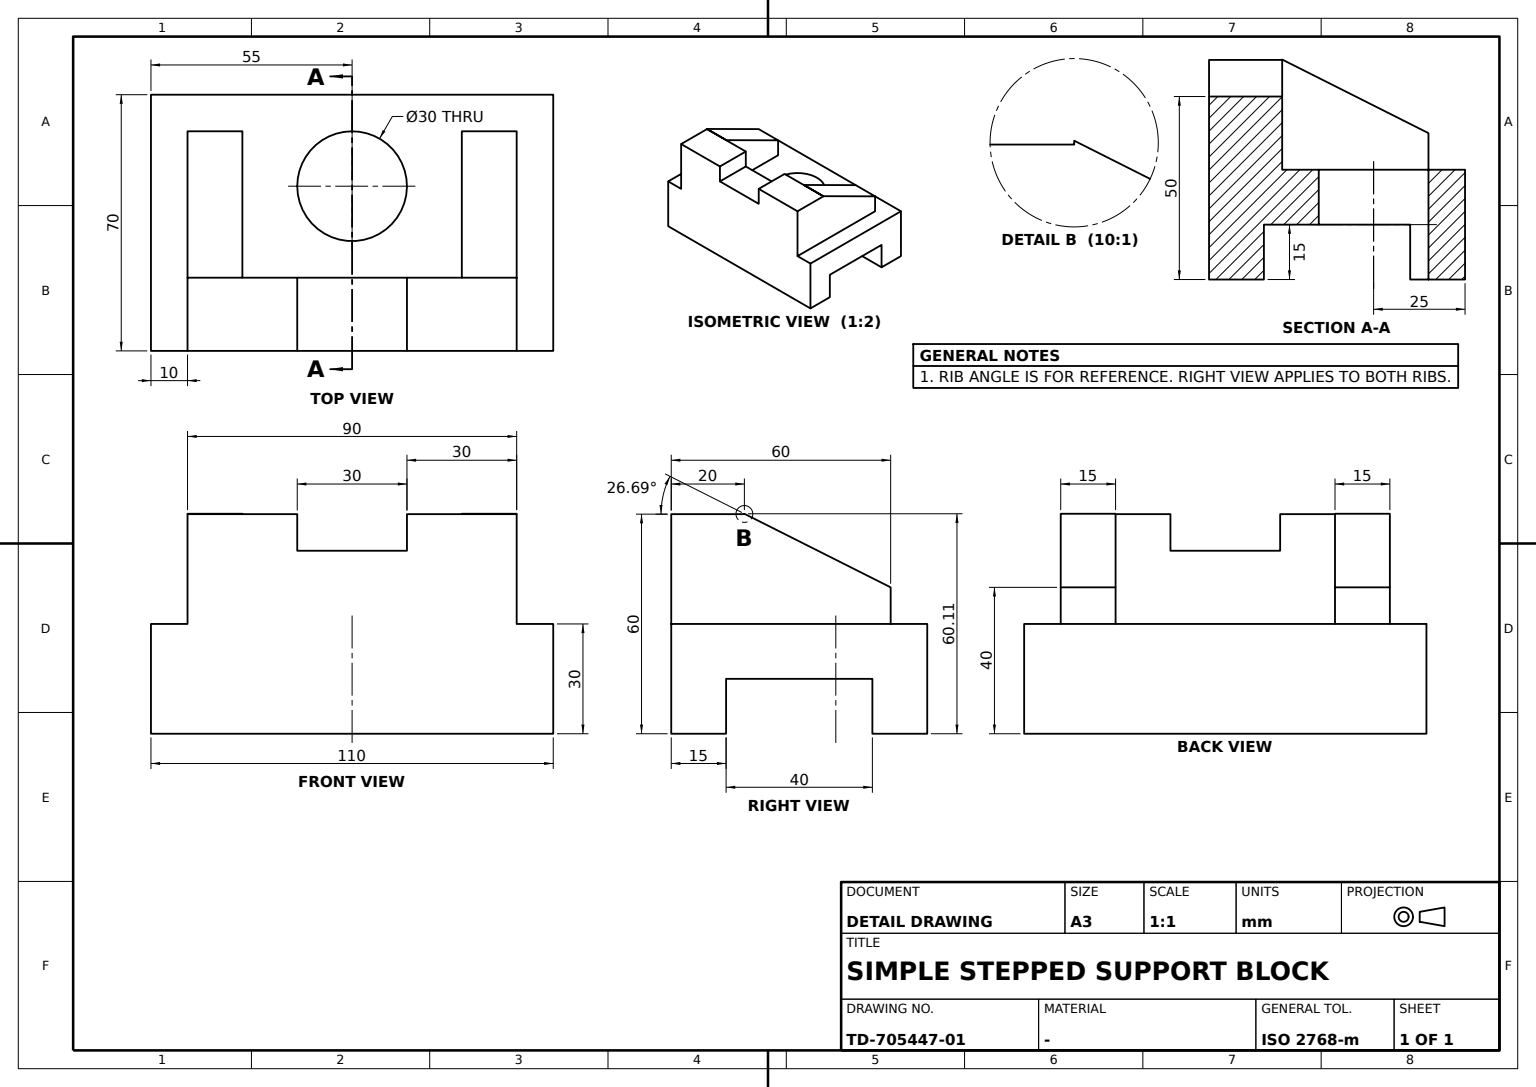
ISO-10303-21;
HEADER;
FILE_DESCRIPTION((''),'2;1');
FILE_NAME('','',(''),(''),'','','');
FILE_SCHEMA(('AUTOMOTIVE_DESIGN'));
ENDSEC;
DATA;
#1=APPLICATION_CONTEXT('');
#2=PRODUCT_CONTEXT('',#1,'mechanical');
#3=PRODUCT('','','',(#2));
#4=PRODUCT_DEFINITION_FORMATION('','',#3);
#5=PRODUCT_DEFINITION_CONTEXT('',#1,'design');
#6=PRODUCT_DEFINITION('','',#4,#5);
#7=PRODUCT_DEFINITION_SHAPE('','',#6);
#8=(LENGTH_UNIT()NAMED_UNIT(*)SI_UNIT(.MILLI.,.METRE.));
#9=(NAMED_UNIT(*)PLANE_ANGLE_UNIT()SI_UNIT($,.RADIAN.));
#10=(NAMED_UNIT(*)SI_UNIT($,.STERADIAN.)SOLID_ANGLE_UNIT());
#11=UNCERTAINTY_MEASURE_WITH_UNIT(LENGTH_MEASURE(0.005),#8,'distance_accuracy_value','');
#12=(GEOMETRIC_REPRESENTATION_CONTEXT(3)GLOBAL_UNCERTAINTY_ASSIGNED_CONTEXT((#11))GLOBAL_UNIT_ASSIGNED_CONTEXT((#8,#9,#10))REPRESENTATION_CONTEXT('',''));
#13=CARTESIAN_POINT('',(-15.,10.,7.5));
#14=VERTEX_POINT('',#13);
#15=CARTESIAN_POINT('',(0.,10.,7.5));
#16=DIRECTION('',(0.,0.,-1.));
#17=DIRECTION('',(-1.,0.,0.));
#18=AXIS2_PLACEMENT_3D('',#15,#16,#17);
#19=CIRCLE('',#18,15.);
#20=EDGE_CURVE('',#14,#14,#19,.T.);
#21=ORIENTED_EDGE('',*,*,#20,.T.);
#22=EDGE_LOOP('',(#21));
#23=FACE_BOUND('',#22,.T.);
#24=CARTESIAN_POINT('',(-55.,-35.,7.5));
#25=VERTEX_POINT('',#24);
#26=CARTESIAN_POINT('',(-45.,-35.,7.5));
#27=VERTEX_POINT('',#26);
#28=CARTESIAN_POINT('',(0.,-35.,7.5));
#29=DIRECTION('',(1.,0.,0.));
#30=VECTOR('',#29,1000.);
#31=LINE('',#28,#30);
#32=EDGE_CURVE('',#25,#27,#31,.T.);
#33=ORIENTED_EDGE('',*,*,#32,.T.);
#34=CARTESIAN_POINT('',(-45.,25.,7.5));
#35=VERTEX_POINT('',#34);
#36=DIRECTION('',(0.,1.,0.));
#37=VECTOR('',#36,1000.);
#38=LINE('',#26,#37);
#39=EDGE_CURVE('',#27,#35,#38,.T.);
#40=ORIENTED_EDGE('',*,*,#39,.T.);
#41=CARTESIAN_POINT('',(-30.,25.,7.5));
#42=VERTEX_POINT('',#41);
#43=CARTESIAN_POINT('',(0.,25.,7.5));
#44=LINE('',#43,#30);
#45=EDGE_CURVE('',#35,#42,#44,.T.);
#46=ORIENTED_EDGE('',*,*,#45,.T.);
#47=CARTESIAN_POINT('',(-30.,-15.,7.5));
#48=VERTEX_POINT('',#47);
#49=CARTESIAN_POINT('',(-30.,-35.,7.5));
#50=DIRECTION('',(0.,-1.,0.));
#51=VECTOR('',#50,1000.);
#52=LINE('',#49,#51);
#53=EDGE_CURVE('',#42,#48,#52,.T.);
#54=ORIENTED_EDGE('',*,*,#53,.T.);
#55=CARTESIAN_POINT('',(30.,-15.,7.5));
#56=VERTEX_POINT('',#55);
#57=CARTESIAN_POINT('',(0.,-15.,7.5));
#58=LINE('',#57,#30);
#59=EDGE_CURVE('',#48,#56,#58,.T.);
#60=ORIENTED_EDGE('',*,*,#59,.T.);
#61=CARTESIAN_POINT('',(30.,25.,7.5));
#62=VERTEX_POINT('',#61);
#63=CARTESIAN_POINT('',(30.,-35.,7.5));
#64=LINE('',#63,#51);
#65=EDGE_CURVE('',#62,#56,#64,.T.);
#66=ORIENTED_EDGE('',*,*,#65,.F.);
#67=CARTESIAN_POINT('',(45.,25.,7.5));
#68=VERTEX_POINT('',#67);
#69=VECTOR('',#17,1000.);
#70=LINE('',#67,#69);
#71=EDGE_CURVE('',#68,#62,#70,.T.);
#72=ORIENTED_EDGE('',*,*,#71,.F.);
#73=CARTESIAN_POINT('',(45.,-35.,7.5));
#74=VERTEX_POINT('',#73);
#75=LINE('',#73,#37);
#76=EDGE_CURVE('',#74,#68,#75,.T.);
#77=ORIENTED_EDGE('',*,*,#76,.F.);
#78=CARTESIAN_POINT('',(55.,-35.,7.5));
#79=VERTEX_POINT('',#78);
#80=EDGE_CURVE('',#74,#79,#31,.T.);
#81=ORIENTED_EDGE('',*,*,#80,.T.);
#82=CARTESIAN_POINT('',(55.,35.,7.5));
#83=VERTEX_POINT('',#82);
#84=CARTESIAN_POINT('',(55.,0.,7.5));
#85=LINE('',#84,#37);
#86=EDGE_CURVE('',#79,#83,#85,.T.);
#87=ORIENTED_EDGE('',*,*,#86,.T.);
#88=CARTESIAN_POINT('',(-55.,35.,7.5));
#89=VERTEX_POINT('',#88);
#90=CARTESIAN_POINT('',(0.,35.,7.5));
#91=LINE('',#90,#30);
#92=EDGE_CURVE('',#89,#83,#91,.T.);
#93=ORIENTED_EDGE('',*,*,#92,.F.);
#94=CARTESIAN_POINT('',(-55.,0.,7.5));
#95=LINE('',#94,#37);
#96=EDGE_CURVE('',#25,#89,#95,.T.);
#97=ORIENTED_EDGE('',*,*,#96,.F.);
#98=EDGE_LOOP('',(#33,#40,#46,#54,#60,#66,#72,#77,#81,#87,#93,#97));
#99=FACE_BOUND('',#98,.T.);
#100=AXIS2_PLACEMENT_3D('',#28,#16,#36);
#101=PLANE('',#100);
#102=ADVANCED_FACE('',(#23,#99),#101,.F.);
#103=CARTESIAN_POINT('',(-15.,-35.,27.5));
#104=VERTEX_POINT('',#103);
#105=CARTESIAN_POINT('',(-15.,-35.,37.5));
#106=VERTEX_POINT('',#105);
#107=CARTESIAN_POINT('',(-15.,-35.,-22.5));
#108=DIRECTION('',(0.,0.,1.));
#109=VECTOR('',#108,1000.);
#110=LINE('',#107,#109);
#111=EDGE_CURVE('',#104,#106,#110,.T.);
#112=ORIENTED_EDGE('',*,*,#111,.F.);
#113=CARTESIAN_POINT('',(-15.,-15.,27.5));
#114=VERTEX_POINT('',#113);
#115=LINE('',#103,#37);
#116=EDGE_CURVE('',#104,#114,#115,.T.);
#117=ORIENTED_EDGE('',*,*,#116,.T.);
#118=CARTESIAN_POINT('',(-15.,-15.,37.5));
#119=VERTEX_POINT('',#118);
#120=LINE('',#113,#109);
#121=EDGE_CURVE('',#114,#119,#120,.T.);
#122=ORIENTED_EDGE('',*,*,#121,.T.);
#123=LINE('',#105,#37);
#124=EDGE_CURVE('',#106,#119,#123,.T.);
#125=ORIENTED_EDGE('',*,*,#124,.F.);
#126=EDGE_LOOP('',(#112,#117,#122,#125));
#127=FACE_BOUND('',#126,.T.);
#128=AXIS2_PLACEMENT_3D('',#103,#17,#108);
#129=PLANE('',#128);
#130=ADVANCED_FACE('',(#127),#129,.F.);
#131=CARTESIAN_POINT('',(-45.,25.,17.5));
#132=VERTEX_POINT('',#131);
#133=CARTESIAN_POINT('',(-30.,25.,17.5));
#134=VERTEX_POINT('',#133);
#135=CARTESIAN_POINT('',(45.,25.,17.5));
#136=LINE('',#135,#30);
#137=EDGE_CURVE('',#132,#134,#136,.T.);
#138=ORIENTED_EDGE('',*,*,#137,.F.);
#139=CARTESIAN_POINT('',(-45.,-15.,37.605849));
#140=VERTEX_POINT('',#139);
#141=DIRECTION('',(0.,0.893479455,-0.449104067));
#142=VECTOR('',#141,1000.);
#143=LINE('',#139,#142);
#144=EDGE_CURVE('',#140,#132,#143,.T.);
#145=ORIENTED_EDGE('',*,*,#144,.F.);
#146=CARTESIAN_POINT('',(-30.,-15.,37.605849));
#147=VERTEX_POINT('',#146);
#148=CARTESIAN_POINT('',(45.,-15.,37.605849));
#149=LINE('',#148,#30);
#150=EDGE_CURVE('',#140,#147,#149,.T.);
#151=ORIENTED_EDGE('',*,*,#150,.T.);
#152=LINE('',#146,#142);
#153=EDGE_CURVE('',#147,#134,#152,.T.);
#154=ORIENTED_EDGE('',*,*,#153,.T.);
#155=EDGE_LOOP('',(#138,#145,#151,#154));
#156=FACE_BOUND('',#155,.T.);
#157=DIRECTION('',(0.,0.449104067,0.893479455));
#158=AXIS2_PLACEMENT_3D('',#148,#157,#141);
#159=PLANE('',#158);
#160=ADVANCED_FACE('',(#156),#159,.T.);
#161=ORIENTED_EDGE('',*,*,#92,.T.);
#162=CARTESIAN_POINT('',(55.,35.,-22.5));
#163=VERTEX_POINT('',#162);
#164=CARTESIAN_POINT('',(55.,35.,0.));
#165=VECTOR('',#16,1000.);
#166=LINE('',#164,#165);
#167=EDGE_CURVE('',#83,#163,#166,.T.);
#168=ORIENTED_EDGE('',*,*,#167,.T.);
#169=CARTESIAN_POINT('',(-55.,35.,-22.5));
#170=VERTEX_POINT('',#169);
#171=CARTESIAN_POINT('',(0.,35.,-22.5));
#172=LINE('',#171,#30);
#173=EDGE_CURVE('',#170,#163,#172,.T.);
#174=ORIENTED_EDGE('',*,*,#173,.F.);
#175=CARTESIAN_POINT('',(-55.,35.,0.));
#176=LINE('',#175,#165);
#177=EDGE_CURVE('',#89,#170,#176,.T.);
#178=ORIENTED_EDGE('',*,*,#177,.F.);
#179=EDGE_LOOP('',(#161,#168,#174,#178));
#180=FACE_BOUND('',#179,.T.);
#181=AXIS2_PLACEMENT_3D('',#90,#50,#16);
#182=PLANE('',#181);
#183=ADVANCED_FACE('',(#180),#182,.F.);
#184=CARTESIAN_POINT('',(-45.,-35.,37.5));
#185=VERTEX_POINT('',#184);
#186=CARTESIAN_POINT('',(-45.,-15.,37.5));
#187=VERTEX_POINT('',#186);
#188=LINE('',#184,#37);
#189=EDGE_CURVE('',#185,#187,#188,.T.);
#190=ORIENTED_EDGE('',*,*,#189,.F.);
#191=CARTESIAN_POINT('',(0.,-35.,37.5));
#192=LINE('',#191,#69);
#193=EDGE_CURVE('',#106,#185,#192,.T.);
#194=ORIENTED_EDGE('',*,*,#193,.F.);
#195=ORIENTED_EDGE('',*,*,#124,.T.);
#196=CARTESIAN_POINT('',(-30.,-15.,37.5));
#197=VERTEX_POINT('',#196);
#198=CARTESIAN_POINT('',(45.,-15.,37.5));
#199=LINE('',#198,#69);
#200=EDGE_CURVE('',#119,#197,#199,.T.);
#201=ORIENTED_EDGE('',*,*,#200,.T.);
#202=EDGE_CURVE('',#197,#187,#199,.T.);
#203=ORIENTED_EDGE('',*,*,#202,.T.);
#204=EDGE_LOOP('',(#190,#194,#195,#201,#203));
#205=FACE_BOUND('',#204,.T.);
#206=CARTESIAN_POINT('',(45.,-35.,37.5));
#207=AXIS2_PLACEMENT_3D('',#206,#16,#17);
#208=PLANE('',#207);
#209=ADVANCED_FACE('',(#205),#208,.F.);
#210=CARTESIAN_POINT('',(55.,-35.,-22.5));
#211=VERTEX_POINT('',#210);
#212=CARTESIAN_POINT('',(55.,-35.,0.));
#213=LINE('',#212,#109);
#214=EDGE_CURVE('',#211,#79,#213,.T.);
#215=ORIENTED_EDGE('',*,*,#214,.F.);
#216=CARTESIAN_POINT('',(55.,-20.,-22.5));
#217=VERTEX_POINT('',#216);
#218=CARTESIAN_POINT('',(55.,0.,-22.5));
#219=LINE('',#218,#51);
#220=EDGE_CURVE('',#217,#211,#219,.T.);
#221=ORIENTED_EDGE('',*,*,#220,.F.);
#222=CARTESIAN_POINT('',(55.,-20.,-7.5));
#223=VERTEX_POINT('',#222);
#224=CARTESIAN_POINT('',(55.,-20.,0.));
#225=LINE('',#224,#165);
#226=EDGE_CURVE('',#223,#217,#225,.T.);
#227=ORIENTED_EDGE('',*,*,#226,.F.);
#228=CARTESIAN_POINT('',(55.,20.,-7.5));
#229=VERTEX_POINT('',#228);
#230=CARTESIAN_POINT('',(55.,0.,-7.5));
#231=LINE('',#230,#51);
#232=EDGE_CURVE('',#229,#223,#231,.T.);
#233=ORIENTED_EDGE('',*,*,#232,.F.);
#234=CARTESIAN_POINT('',(55.,20.,-22.5));
#235=VERTEX_POINT('',#234);
#236=CARTESIAN_POINT('',(55.,20.,0.));
#237=LINE('',#236,#109);
#238=EDGE_CURVE('',#235,#229,#237,.T.);
#239=ORIENTED_EDGE('',*,*,#238,.F.);
#240=EDGE_CURVE('',#163,#235,#219,.T.);
#241=ORIENTED_EDGE('',*,*,#240,.F.);
#242=ORIENTED_EDGE('',*,*,#167,.F.);
#243=ORIENTED_EDGE('',*,*,#86,.F.);
#244=EDGE_LOOP('',(#215,#221,#227,#233,#239,#241,#242,#243));
#245=FACE_BOUND('',#244,.T.);
#246=CARTESIAN_POINT('',(55.,0.,0.));
#247=AXIS2_PLACEMENT_3D('',#246,#29,#36);
#248=PLANE('',#247);
#249=ADVANCED_FACE('',(#245),#248,.T.);
#250=ORIENTED_EDGE('',*,*,#238,.T.);
#251=CARTESIAN_POINT('',(11.18034,20.,-7.5));
#252=VERTEX_POINT('',#251);
#253=CARTESIAN_POINT('',(0.,20.,-7.5));
#254=LINE('',#253,#30);
#255=EDGE_CURVE('',#252,#229,#254,.T.);
#256=ORIENTED_EDGE('',*,*,#255,.F.);
#257=CARTESIAN_POINT('',(11.18034,20.,-22.5));
#258=VERTEX_POINT('',#257);
#259=LINE('',#257,#165);
#260=EDGE_CURVE('',#258,#252,#259,.F.);
#261=ORIENTED_EDGE('',*,*,#260,.F.);
#262=CARTESIAN_POINT('',(0.,20.,-22.5));
#263=LINE('',#262,#30);
#264=EDGE_CURVE('',#258,#235,#263,.T.);
#265=ORIENTED_EDGE('',*,*,#264,.T.);
#266=EDGE_LOOP('',(#250,#256,#261,#265));
#267=FACE_BOUND('',#266,.T.);
#268=AXIS2_PLACEMENT_3D('',#262,#36,#108);
#269=PLANE('',#268);
#270=ADVANCED_FACE('',(#267),#269,.F.);
#271=CARTESIAN_POINT('',(15.,-35.,27.5));
#272=VERTEX_POINT('',#271);
#273=CARTESIAN_POINT('',(15.,-15.,27.5));
#274=VERTEX_POINT('',#273);
#275=LINE('',#271,#37);
#276=EDGE_CURVE('',#272,#274,#275,.T.);
#277=ORIENTED_EDGE('',*,*,#276,.T.);
#278=LINE('',#273,#69);
#279=EDGE_CURVE('',#274,#114,#278,.T.);
#280=ORIENTED_EDGE('',*,*,#279,.T.);
#281=ORIENTED_EDGE('',*,*,#116,.F.);
#282=CARTESIAN_POINT('',(0.,-35.,27.5));
#283=LINE('',#282,#69);
#284=EDGE_CURVE('',#272,#104,#283,.T.);
#285=ORIENTED_EDGE('',*,*,#284,.F.);
#286=EDGE_LOOP('',(#277,#280,#281,#285));
#287=FACE_BOUND('',#286,.T.);
#288=AXIS2_PLACEMENT_3D('',#271,#16,#17);
#289=PLANE('',#288);
#290=ADVANCED_FACE('',(#287),#289,.F.);
#291=CARTESIAN_POINT('',(30.,-15.,37.5));
#292=VERTEX_POINT('',#291);
#293=CARTESIAN_POINT('',(30.,-15.,37.605849));
#294=VERTEX_POINT('',#293);
#295=CARTESIAN_POINT('',(30.,-15.,0.));
#296=LINE('',#295,#109);
#297=EDGE_CURVE('',#292,#294,#296,.T.);
#298=ORIENTED_EDGE('',*,*,#297,.T.);
#299=CARTESIAN_POINT('',(30.,25.,17.5));
#300=VERTEX_POINT('',#299);
#301=LINE('',#293,#142);
#302=EDGE_CURVE('',#294,#300,#301,.T.);
#303=ORIENTED_EDGE('',*,*,#302,.T.);
#304=LINE('',#299,#165);
#305=EDGE_CURVE('',#300,#62,#304,.T.);
#306=ORIENTED_EDGE('',*,*,#305,.T.);
#307=ORIENTED_EDGE('',*,*,#65,.T.);
#308=EDGE_CURVE('',#56,#292,#296,.T.);
#309=ORIENTED_EDGE('',*,*,#308,.T.);
#310=EDGE_LOOP('',(#298,#303,#306,#307,#309));
#311=FACE_BOUND('',#310,.T.);
#312=CARTESIAN_POINT('',(30.,0.,0.));
#313=AXIS2_PLACEMENT_3D('',#312,#29,#36);
#314=PLANE('',#313);
#315=ADVANCED_FACE('',(#311),#314,.F.);
#316=VERTEX_POINT('',#135);
#317=LINE('',#135,#69);
#318=EDGE_CURVE('',#316,#300,#317,.T.);
#319=ORIENTED_EDGE('',*,*,#318,.T.);
#320=ORIENTED_EDGE('',*,*,#302,.F.);
#321=VERTEX_POINT('',#148);
#322=CARTESIAN_POINT('',(0.,-15.,37.605849));
#323=LINE('',#322,#69);
#324=EDGE_CURVE('',#321,#294,#323,.T.);
#325=ORIENTED_EDGE('',*,*,#324,.F.);
#326=CARTESIAN_POINT('',(45.,-18.88568,39.558971));
#327=LINE('',#326,#142);
#328=EDGE_CURVE('',#321,#316,#327,.T.);
#329=ORIENTED_EDGE('',*,*,#328,.T.);
#330=EDGE_LOOP('',(#319,#320,#325,#329));
#331=FACE_BOUND('',#330,.T.);
#332=ADVANCED_FACE('',(#331),#159,.T.);
#333=ORIENTED_EDGE('',*,*,#189,.T.);
#334=CARTESIAN_POINT('',(-45.,-15.,0.));
#335=LINE('',#334,#109);
#336=EDGE_CURVE('',#187,#140,#335,.T.);
#337=ORIENTED_EDGE('',*,*,#336,.T.);
#338=ORIENTED_EDGE('',*,*,#144,.T.);
#339=LINE('',#131,#165);
#340=EDGE_CURVE('',#132,#35,#339,.T.);
#341=ORIENTED_EDGE('',*,*,#340,.T.);
#342=ORIENTED_EDGE('',*,*,#39,.F.);
#343=CARTESIAN_POINT('',(-45.,-35.,-22.5));
#344=LINE('',#343,#165);
#345=EDGE_CURVE('',#185,#27,#344,.T.);
#346=ORIENTED_EDGE('',*,*,#345,.F.);
#347=EDGE_LOOP('',(#333,#337,#338,#341,#342,#346));
#348=FACE_BOUND('',#347,.T.);
#349=AXIS2_PLACEMENT_3D('',#184,#29,#16);
#350=PLANE('',#349);
#351=ADVANCED_FACE('',(#348),#350,.F.);
#352=CARTESIAN_POINT('',(-11.18034,20.,-7.5));
#353=VERTEX_POINT('',#352);
#354=CARTESIAN_POINT('',(0.,10.,-7.5));
#355=AXIS2_PLACEMENT_3D('',#354,#108,#29);
#356=CIRCLE('',#355,15.);
#357=EDGE_CURVE('',#353,#252,#356,.T.);
#358=ORIENTED_EDGE('',*,*,#357,.T.);
#359=ORIENTED_EDGE('',*,*,#255,.T.);
#360=ORIENTED_EDGE('',*,*,#232,.T.);
#361=CARTESIAN_POINT('',(-55.,-20.,-7.5));
#362=VERTEX_POINT('',#361);
#363=CARTESIAN_POINT('',(0.,-20.,-7.5));
#364=LINE('',#363,#30);
#365=EDGE_CURVE('',#362,#223,#364,.T.);
#366=ORIENTED_EDGE('',*,*,#365,.F.);
#367=CARTESIAN_POINT('',(-55.,20.,-7.5));
#368=VERTEX_POINT('',#367);
#369=CARTESIAN_POINT('',(-55.,0.,-7.5));
#370=LINE('',#369,#51);
#371=EDGE_CURVE('',#368,#362,#370,.T.);
#372=ORIENTED_EDGE('',*,*,#371,.F.);
#373=EDGE_CURVE('',#368,#353,#254,.T.);
#374=ORIENTED_EDGE('',*,*,#373,.T.);
#375=EDGE_LOOP('',(#358,#359,#360,#366,#372,#374));
#376=FACE_BOUND('',#375,.T.);
#377=AXIS2_PLACEMENT_3D('',#253,#108,#50);
#378=PLANE('',#377);
#379=ADVANCED_FACE('',(#376),#378,.F.);
#380=ORIENTED_EDGE('',*,*,#193,.T.);
#381=ORIENTED_EDGE('',*,*,#345,.T.);
#382=ORIENTED_EDGE('',*,*,#32,.F.);
#383=CARTESIAN_POINT('',(-55.,-35.,-22.5));
#384=VERTEX_POINT('',#383);
#385=CARTESIAN_POINT('',(-55.,-35.,0.));
#386=LINE('',#385,#109);
#387=EDGE_CURVE('',#384,#25,#386,.T.);
#388=ORIENTED_EDGE('',*,*,#387,.F.);
#389=CARTESIAN_POINT('',(0.,-35.,-22.5));
#390=LINE('',#389,#30);
#391=EDGE_CURVE('',#384,#211,#390,.T.);
#392=ORIENTED_EDGE('',*,*,#391,.T.);
#393=ORIENTED_EDGE('',*,*,#214,.T.);
#394=ORIENTED_EDGE('',*,*,#80,.F.);
#395=VERTEX_POINT('',#206);
#396=CARTESIAN_POINT('',(45.,-35.,-22.5));
#397=LINE('',#396,#109);
#398=EDGE_CURVE('',#74,#395,#397,.T.);
#399=ORIENTED_EDGE('',*,*,#398,.T.);
#400=CARTESIAN_POINT('',(15.,-35.,37.5));
#401=VERTEX_POINT('',#400);
#402=EDGE_CURVE('',#395,#401,#192,.T.);
#403=ORIENTED_EDGE('',*,*,#402,.T.);
#404=CARTESIAN_POINT('',(15.,-35.,-22.5));
#405=LINE('',#404,#165);
#406=EDGE_CURVE('',#401,#272,#405,.T.);
#407=ORIENTED_EDGE('',*,*,#406,.T.);
#408=ORIENTED_EDGE('',*,*,#284,.T.);
#409=ORIENTED_EDGE('',*,*,#111,.T.);
#410=EDGE_LOOP('',(#380,#381,#382,#388,#392,#393,#394,#399,#403,#407,#408,#409));
#411=FACE_BOUND('',#410,.T.);
#412=AXIS2_PLACEMENT_3D('',#389,#36,#108);
#413=PLANE('',#412);
#414=ADVANCED_FACE('',(#411),#413,.F.);
#415=ORIENTED_EDGE('',*,*,#365,.T.);
#416=ORIENTED_EDGE('',*,*,#226,.T.);
#417=CARTESIAN_POINT('',(-55.,-20.,-22.5));
#418=VERTEX_POINT('',#417);
#419=CARTESIAN_POINT('',(0.,-20.,-22.5));
#420=LINE('',#419,#30);
#421=EDGE_CURVE('',#418,#217,#420,.T.);
#422=ORIENTED_EDGE('',*,*,#421,.F.);
#423=CARTESIAN_POINT('',(-55.,-20.,0.));
#424=LINE('',#423,#165);
#425=EDGE_CURVE('',#362,#418,#424,.T.);
#426=ORIENTED_EDGE('',*,*,#425,.F.);
#427=EDGE_LOOP('',(#415,#416,#422,#426));
#428=FACE_BOUND('',#427,.T.);
#429=AXIS2_PLACEMENT_3D('',#363,#50,#16);
#430=PLANE('',#429);
#431=ADVANCED_FACE('',(#428),#430,.F.);
#432=LINE('',#67,#165);
#433=EDGE_CURVE('',#316,#68,#432,.T.);
#434=ORIENTED_EDGE('',*,*,#433,.F.);
#435=ORIENTED_EDGE('',*,*,#328,.F.);
#436=VERTEX_POINT('',#198);
#437=CARTESIAN_POINT('',(45.,-15.,7.5));
#438=LINE('',#437,#109);
#439=EDGE_CURVE('',#436,#321,#438,.T.);
#440=ORIENTED_EDGE('',*,*,#439,.F.);
#441=LINE('',#206,#37);
#442=EDGE_CURVE('',#395,#436,#441,.T.);
#443=ORIENTED_EDGE('',*,*,#442,.F.);
#444=ORIENTED_EDGE('',*,*,#398,.F.);
#445=ORIENTED_EDGE('',*,*,#76,.T.);
#446=EDGE_LOOP('',(#434,#435,#440,#443,#444,#445));
#447=FACE_BOUND('',#446,.T.);
#448=AXIS2_PLACEMENT_3D('',#73,#17,#108);
#449=PLANE('',#448);
#450=ADVANCED_FACE('',(#447),#449,.F.);
#451=CARTESIAN_POINT('',(15.,-15.,37.5));
#452=VERTEX_POINT('',#451);
#453=LINE('',#451,#165);
#454=EDGE_CURVE('',#452,#274,#453,.T.);
#455=ORIENTED_EDGE('',*,*,#454,.T.);
#456=ORIENTED_EDGE('',*,*,#276,.F.);
#457=ORIENTED_EDGE('',*,*,#406,.F.);
#458=LINE('',#400,#37);
#459=EDGE_CURVE('',#401,#452,#458,.T.);
#460=ORIENTED_EDGE('',*,*,#459,.T.);
#461=EDGE_LOOP('',(#455,#456,#457,#460));
#462=FACE_BOUND('',#461,.T.);
#463=AXIS2_PLACEMENT_3D('',#400,#29,#16);
#464=PLANE('',#463);
#465=ADVANCED_FACE('',(#462),#464,.F.);
#466=CARTESIAN_POINT('',(-11.18034,20.,-22.5));
#467=VERTEX_POINT('',#466);
#468=LINE('',#466,#165);
#469=EDGE_CURVE('',#353,#467,#468,.T.);
#470=ORIENTED_EDGE('',*,*,#469,.T.);
#471=CARTESIAN_POINT('',(0.,10.,-22.5));
#472=AXIS2_PLACEMENT_3D('',#471,#108,#29);
#473=CIRCLE('',#472,15.);
#474=EDGE_CURVE('',#258,#467,#473,.T.);
#475=ORIENTED_EDGE('',*,*,#474,.F.);
#476=ORIENTED_EDGE('',*,*,#260,.T.);
#477=ORIENTED_EDGE('',*,*,#357,.F.);
#478=EDGE_LOOP('',(#470,#475,#476,#477));
#479=FACE_BOUND('',#478,.T.);
#480=ORIENTED_EDGE('',*,*,#20,.F.);
#481=EDGE_LOOP('',(#480));
#482=FACE_BOUND('',#481,.T.);
#483=CARTESIAN_POINT('',(0.,10.,7.4));
#484=AXIS2_PLACEMENT_3D('',#483,#16,#29);
#485=CYLINDRICAL_SURFACE('',#484,15.);
#486=ADVANCED_FACE('',(#479,#482),#485,.F.);
#487=EDGE_CURVE('',#436,#292,#199,.T.);
#488=ORIENTED_EDGE('',*,*,#487,.T.);
#489=EDGE_CURVE('',#292,#452,#199,.T.);
#490=ORIENTED_EDGE('',*,*,#489,.T.);
#491=ORIENTED_EDGE('',*,*,#459,.F.);
#492=ORIENTED_EDGE('',*,*,#402,.F.);
#493=ORIENTED_EDGE('',*,*,#442,.T.);
#494=EDGE_LOOP('',(#488,#490,#491,#492,#493));
#495=FACE_BOUND('',#494,.T.);
#496=ADVANCED_FACE('',(#495),#208,.F.);
#497=ORIENTED_EDGE('',*,*,#433,.T.);
#498=ORIENTED_EDGE('',*,*,#71,.T.);
#499=ORIENTED_EDGE('',*,*,#305,.F.);
#500=ORIENTED_EDGE('',*,*,#318,.F.);
#501=EDGE_LOOP('',(#497,#498,#499,#500));
#502=FACE_BOUND('',#501,.T.);
#503=AXIS2_PLACEMENT_3D('',#135,#36,#16);
#504=PLANE('',#503);
#505=ADVANCED_FACE('',(#502),#504,.T.);
#506=CARTESIAN_POINT('',(-30.,-15.,0.));
#507=LINE('',#506,#109);
#508=EDGE_CURVE('',#197,#147,#507,.T.);
#509=ORIENTED_EDGE('',*,*,#508,.T.);
#510=ORIENTED_EDGE('',*,*,#150,.F.);
#511=ORIENTED_EDGE('',*,*,#336,.F.);
#512=ORIENTED_EDGE('',*,*,#202,.F.);
#513=EDGE_LOOP('',(#509,#510,#511,#512));
#514=FACE_BOUND('',#513,.T.);
#515=CARTESIAN_POINT('',(0.,-15.,0.));
#516=AXIS2_PLACEMENT_3D('',#515,#50,#29);
#517=PLANE('',#516);
#518=ADVANCED_FACE('',(#514),#517,.T.);
#519=CARTESIAN_POINT('',(-55.,20.,-22.5));
#520=VERTEX_POINT('',#519);
#521=CARTESIAN_POINT('',(-55.,0.,-22.5));
#522=LINE('',#521,#51);
#523=EDGE_CURVE('',#170,#520,#522,.T.);
#524=ORIENTED_EDGE('',*,*,#523,.T.);
#525=CARTESIAN_POINT('',(-55.,20.,0.));
#526=LINE('',#525,#109);
#527=EDGE_CURVE('',#520,#368,#526,.T.);
#528=ORIENTED_EDGE('',*,*,#527,.T.);
#529=ORIENTED_EDGE('',*,*,#371,.T.);
#530=ORIENTED_EDGE('',*,*,#425,.T.);
#531=EDGE_CURVE('',#418,#384,#522,.T.);
#532=ORIENTED_EDGE('',*,*,#531,.T.);
#533=ORIENTED_EDGE('',*,*,#387,.T.);
#534=ORIENTED_EDGE('',*,*,#96,.T.);
#535=ORIENTED_EDGE('',*,*,#177,.T.);
#536=EDGE_LOOP('',(#524,#528,#529,#530,#532,#533,#534,#535));
#537=FACE_BOUND('',#536,.T.);
#538=CARTESIAN_POINT('',(-55.,0.,0.));
#539=AXIS2_PLACEMENT_3D('',#538,#29,#36);
#540=PLANE('',#539);
#541=ADVANCED_FACE('',(#537),#540,.F.);
#542=ORIENTED_EDGE('',*,*,#121,.F.);
#543=ORIENTED_EDGE('',*,*,#279,.F.);
#544=ORIENTED_EDGE('',*,*,#454,.F.);
#545=ORIENTED_EDGE('',*,*,#489,.F.);
#546=ORIENTED_EDGE('',*,*,#308,.F.);
#547=ORIENTED_EDGE('',*,*,#59,.F.);
#548=EDGE_CURVE('',#48,#197,#507,.T.);
#549=ORIENTED_EDGE('',*,*,#548,.T.);
#550=ORIENTED_EDGE('',*,*,#200,.F.);
#551=EDGE_LOOP('',(#542,#543,#544,#545,#546,#547,#549,#550));
#552=FACE_BOUND('',#551,.T.);
#553=ADVANCED_FACE('',(#552),#517,.F.);
#554=ORIENTED_EDGE('',*,*,#474,.T.);
#555=EDGE_CURVE('',#520,#467,#263,.T.);
#556=ORIENTED_EDGE('',*,*,#555,.F.);
#557=ORIENTED_EDGE('',*,*,#523,.F.);
#558=ORIENTED_EDGE('',*,*,#173,.T.);
#559=ORIENTED_EDGE('',*,*,#240,.T.);
#560=ORIENTED_EDGE('',*,*,#264,.F.);
#561=EDGE_LOOP('',(#554,#556,#557,#558,#559,#560));
#562=FACE_BOUND('',#561,.T.);
#563=AXIS2_PLACEMENT_3D('',#171,#108,#50);
#564=PLANE('',#563);
#565=ADVANCED_FACE('',(#562),#564,.F.);
#566=ORIENTED_EDGE('',*,*,#324,.T.);
#567=ORIENTED_EDGE('',*,*,#297,.F.);
#568=ORIENTED_EDGE('',*,*,#487,.F.);
#569=ORIENTED_EDGE('',*,*,#439,.T.);
#570=EDGE_LOOP('',(#566,#567,#568,#569));
#571=FACE_BOUND('',#570,.T.);
#572=ADVANCED_FACE('',(#571),#517,.T.);
#573=ORIENTED_EDGE('',*,*,#531,.F.);
#574=ORIENTED_EDGE('',*,*,#421,.T.);
#575=ORIENTED_EDGE('',*,*,#220,.T.);
#576=ORIENTED_EDGE('',*,*,#391,.F.);
#577=EDGE_LOOP('',(#573,#574,#575,#576));
#578=FACE_BOUND('',#577,.T.);
#579=ADVANCED_FACE('',(#578),#564,.F.);
#580=ORIENTED_EDGE('',*,*,#469,.F.);
#581=ORIENTED_EDGE('',*,*,#373,.F.);
#582=ORIENTED_EDGE('',*,*,#527,.F.);
#583=ORIENTED_EDGE('',*,*,#555,.T.);
#584=EDGE_LOOP('',(#580,#581,#582,#583));
#585=FACE_BOUND('',#584,.T.);
#586=ADVANCED_FACE('',(#585),#269,.F.);
#587=LINE('',#133,#165);
#588=EDGE_CURVE('',#134,#42,#587,.T.);
#589=ORIENTED_EDGE('',*,*,#588,.T.);
#590=ORIENTED_EDGE('',*,*,#45,.F.);
#591=ORIENTED_EDGE('',*,*,#340,.F.);
#592=ORIENTED_EDGE('',*,*,#137,.T.);
#593=EDGE_LOOP('',(#589,#590,#591,#592));
#594=FACE_BOUND('',#593,.T.);
#595=ADVANCED_FACE('',(#594),#504,.T.);
#596=ORIENTED_EDGE('',*,*,#53,.F.);
#597=ORIENTED_EDGE('',*,*,#588,.F.);
#598=ORIENTED_EDGE('',*,*,#153,.F.);
#599=ORIENTED_EDGE('',*,*,#508,.F.);
#600=ORIENTED_EDGE('',*,*,#548,.F.);
#601=EDGE_LOOP('',(#596,#597,#598,#599,#600));
#602=FACE_BOUND('',#601,.T.);
#603=CARTESIAN_POINT('',(-30.,0.,0.));
#604=AXIS2_PLACEMENT_3D('',#603,#29,#36);
#605=PLANE('',#604);
#606=ADVANCED_FACE('',(#602),#605,.T.);
#607=CLOSED_SHELL('',(#102,#130,#160,#183,#209,#249,#270,#290,#315,#332,#351,#379,#414,#431,#450,#465,#486,#496,#505,#518,#541,#553,#565,#572,#579,#586,#595,#606));
#608=MANIFOLD_SOLID_BREP('',#607);
#609=ADVANCED_BREP_SHAPE_REPRESENTATION('',(#608),#12);
#610=SHAPE_DEFINITION_REPRESENTATION(#7,#609);
ENDSEC;
END-ISO-10303-21;
